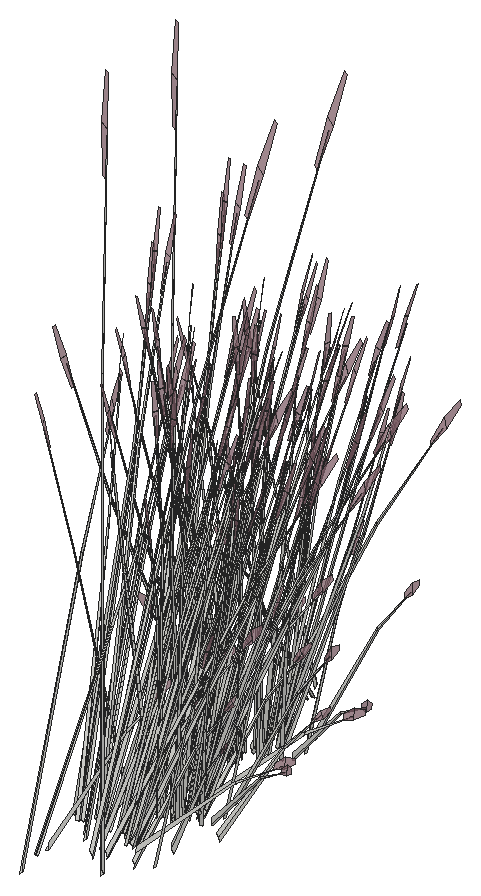
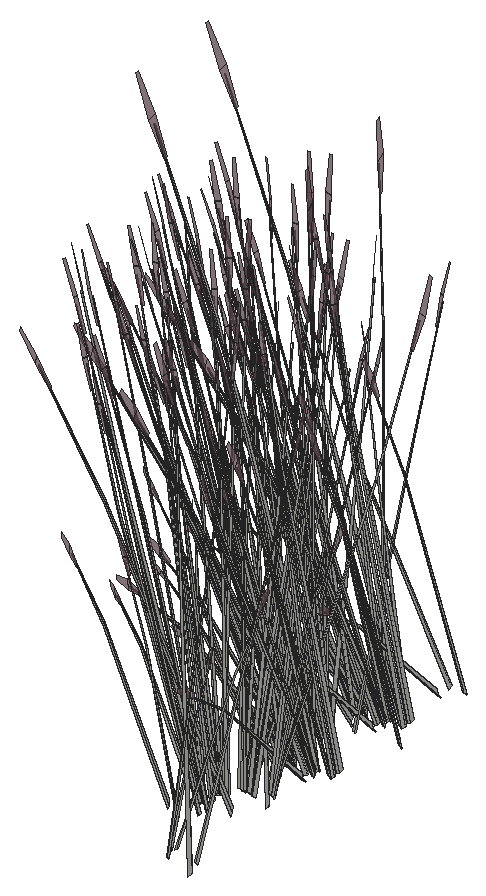
# SketchUp Ruby script. Lengths in inches.
U = 1.inch
M = Sketchup.active_model
def pt(a) = Geom::Point3d.new(a.map { |v| v * U })
def face(e, loops, mat)
  f = e.add_face(loops[0].map { |a| pt(a) })
  loops[1..].each { |l| e.add_face(l.map { |a| pt(a) }).erase! }
  f.material = f.back_material = mat if mat
  f
end
# faces: each face lists its corners as indices into pts; further lists are holes
def faces(e, pts, list, mat = nil) = list.each { |f| face(e, (f[0].is_a?(Array) ? f : [f]).map { |l| l.map { |i| pts[i] } }, mat) }
# xy, xz, yz: faces in a plane at the given z, y or x. An outline is a flat list of corners, or four numbers for a rectangle; further outlines are holes
def ring(l) = l.size == 4 ? [[l[0], l[1]], [l[2], l[1]], [l[2], l[3]], [l[0], l[3]]] : l.each_slice(2).to_a
def flat(e, list, mat, &to3) = list.each { |f| face(e, (f[0].is_a?(Array) ? f : [f]).map { |l| ring(l).map { |u, v| to3.(u, v) } }, mat) }
def xy(e, z, list, mat = nil) = flat(e, list, mat) { |x, y| [x, y, z] }
def xz(e, y, list, mat = nil) = flat(e, list, mat) { |x, z| [x, y, z] }
def yz(e, x, list, mat = nil) = flat(e, list, mat) { |y, z| [x, y, z] }
def lines(e, pts, list) = list.each { |a, b| e.add_line(pt(pts[a]), pt(pts[b])) }
# prism: a flat outline (further loops are holes) pulled along v
def prism(e, loops, v, mat = nil)
  f = face(e, loops, mat); d = Geom::Vector3d.new(v.map { |x| x * U })
  f.pushpull(f.normal.samedirection?(d) ? d.length : -d.length)
end
def box(e, o, s, mat = nil) = prism(e, [[o, [o[0] + s[0], o[1], o[2]], [o[0] + s[0], o[1] + s[1], o[2]], [o[0], o[1] + s[1], o[2]]]], [0, 0, s[2]], mat)
def at(x, y, z, deg = 0) = Geom::Transformation.translation(pt([x, y, z])) * Geom::Transformation.rotation(ORIGIN, Z_AXIS, deg.degrees)
def axes(o, x, y, z) = Geom::Transformation.new([*x, 0, *y, 0, *z, 0, *pt(o).to_a, 1])
def part(name) = M.definitions.add(name)
# library, detail: a bought-in or finely detailed component or shape, given as its bounding box
def library(name, o, s) = part(name).tap { |d| box(d.entities, o, s) }
def detail(e, o, s) = box(e.add_group.entities, o, s)
def put(e, d, t, mat = nil) = e.add_instance(d, t).tap { |i| i.material = mat if mat }
def group(e, t, mat = nil) = e.add_group.tap { |g| g.transformation = t; g.material = mat if mat }.entities
root = M.entities
M.materials.add("LightPink_Translucent").color = [144, 107, 117]
M.materials["LightPink_Translucent"].alpha = 0.75
c1 = part("blade")
p = [[2.15,0.21,22],[0,0.17,0],[0.09,0.45,0],[2.18,0.31,22],[2.29,0.31,22],[0.38,0.45,0],
  [2.48,0.24,33],[2.49,0.24,33],[2.48,0.22,33]]
faces(c1.entities,p,[[0,1,2,3],[4,5,2,3],[6,3,4,7],[8,0,3,6]])
c2 = part("seeds")
p = [[0.3,-0.1,1.38],[-0.01,-0.03,1.59],[-0.01,-0.03,0.03],[0.14,-0.07,-0.07],[0.29,-0.03,3],[0.15,0.01,3.11]]
faces(c2.entities,p,[[0,1,2,3],[1,0,4,5]],"LightPink_Translucent")
c3 = part("blade with seeds")
put(c3.entities,c1,at(0,0,0))
put(c3.entities,c2,axes([2.4,0.25,30.99],[1.5799,-0.05474,1.17369],[-0.12525,1.92788,0.29478],[-0.07173,-0.02425,1.56792]))
put(root,c3,axes([691.71,317.27,267.26],[-0.12452,-0.47997,-0.02898],[0.58854,-0.11034,-0.1314],[0.1229,0.03043,0.43341]))
put(root,c3,axes([690.1875,317.26,268.18],[0.03484,-0.58066,-0.10093],[0.65957,0.01587,-0.56021],[0.25402,0.04034,0.85122]))
put(root,c3,axes([690.09,317.03,268.19],[-0.37017,-0.35748,0.29394],[0.42268,-0.3384,-0.37948],[0.21476,0.05149,0.72609]))
put(root,c3,axes([686.65,312.02,267.22],[-0.01592,-0.21915,1.42242],[0.69015,0.14538,0.11501],[-0.04269,0.3123,0.60807]))
put(root,c3,axes([688.15,320.03,268.19],[-0.19614,0.43908,0.29394],[-0.57222,-0.12807,-0.37948],[-0.05247,-0.17678,0.72609]))
put(root,c3,axes([689.61,320.21,267.93],[0.46327,0.38957,0.39842],[-0.49199,0.33598,0.32852],[0.08546,-0.18277,0.82444]))
put(root,c3,axes([689.78,320.25,267.93],[0.53464,0.0266,0.05337],[-0.01466,0.40172,0.42015],[0.05594,-0.15388,0.64067]))
put(root,c3,axes([687.27,312.85,268.13],[0.31051,0.46426,-0.58968],[-0.63919,0.25873,0.07116],[0.07261,0.22432,0.83415]))
put(root,c3,axes([689.38,320.52,268.19],[-0.4402,0.30062,0.29394],[-0.41671,-0.34326,-0.37948],[0.0634,-0.1744,0.72609]))
put(root,c3,axes([690.16,321.33,268.13],[0.33983,-0.45051,-0.58968],[0.59551,0.32017,0.07116],[0.20291,-0.16322,0.83415]))
put(root,c3,axes([690.14,321.12,267.89],[-0.16713,-0.52135,-0.42412],[0.63294,-0.0912,-0.32852],[0.18138,-0.14003,0.81151]))
put(root,c3,axes([686.8,314.02,267.91],[0.08247,0.09194,1.45204],[0.66552,0.03612,-0.22964],[0.06692,0.20277,0.11645]))
put(root,c3,axes([690.76,316.91,267.91],[0.13956,-0.00966,1.45204],[0.38281,-0.44358,-0.22964],[0.24825,0.05855,0.11645]))
put(root,c3,axes([690.44,321.5,268.18],[-0.60181,-0.31483,-0.10093],[0.34671,-0.45593,-0.56021],[0.17003,-0.15849,0.85122]))
put(root,c3,axes([690.22,316.98,268.13],[0.65035,0.01375,-0.58968],[-0.04368,0.5789,0.07116],[0.27552,0.06109,0.83415]))
put(root,c3,axes([691.92,321.36,267.91],[-0.08498,-0.00434,1.47228],[-0.35287,-0.46464,-0.13912],[0.14171,-0.15278,0.26054]))
put(root,c3,axes([690.92,320.09,266.3],[-0.2167,0.29065,0.95334],[-0.18626,-0.3905,0.70045],[0.17898,-0.09785,0.20998]))
put(root,c3,axes([690.61,317.22,267.76],[0.37017,0.35748,-0.29394],[-0.42268,0.3384,0.37948],[0.21476,0.05149,0.72609]))
put(root,c3,axes([690.42,317.35,267.93],[-0.03276,0.43418,0.05337],[-0.49468,-0.0119,0.42015],[0.18949,0.04543,0.64067]))
put(root,c3,axes([690.61,321.18,267.76],[0.56631,-0.0816,-0.29394],[0.14954,0.46647,0.37948],[0.16229,-0.12529,0.72609]))
put(root,c3,axes([690.47,317.22,267.93],[-0.47971,0.37622,0.39842],[-0.41372,-0.39954,0.32852],[0.22506,0.0694,0.82444]))
put(root,c3,axes([690.15,321.45,268.19],[-0.56631,0.0816,0.29394],[-0.14954,-0.46647,-0.37948],[0.16229,-0.12529,0.72609]))
put(root,c3,axes([688.94,317.65,268.19],[-0.10048,-0.4599,0.29394],[0.5744,-0.12144,-0.37948],[0.15428,0.13179,0.72609]))
put(root,c3,axes([689.28,316.3,267.22],[-0.24166,-0.09837,1.42242],[0.50011,-0.41269,0.11501],[0.3117,0.18617,0.60807]))
put(root,c3,axes([689.33,315.01,267.71],[-0.56218,-0.29666,1.14775],[0.59361,-0.46189,0.49522],[0.18138,0.27836,1.10941]))
put(root,c3,axes([690.18,317.42,266.3],[-0.36631,-0.16417,0.95334],[0.47299,-0.16681,0.70045],[0.12758,0.1413,0.20998]))
put(root,c3,axes([688.89,317.89,268.18],[0.38768,-0.48872,-0.10093],[0.56143,0.28156,-0.56021],[0.19516,0.13808,0.85122]))
put(root,c3,axes([690.66,321.38,267.93],[0.44663,0.24013,0.05337],[-0.26003,0.34195,0.42015],[0.14319,-0.11055,0.64067]))
put(root,c3,axes([690.54,321.28,267.93],[0.16135,0.52549,0.39842],[-0.63294,0.0912,0.32852],[0.18654,-0.12359,0.82444]))
put(root,c3,axes([692.24,321.91,267.91],[0.09028,-0.08697,1.45204],[-0.11555,-0.53348,-0.22964],[0.22652,-0.10115,0.11645]))
put(root,c3,axes([686.33,317.23,268.19],[0.4402,-0.30062,0.29394],[0.41671,0.34326,-0.37948],[-0.0634,0.1744,0.72609]))
put(root,c3,axes([688.38,318.29,267.91],[0.00193,-0.06913,1.47228],[0.55753,-0.30498,-0.13912],[0.19366,0.10886,0.26054]))
put(root,c3,axes([689.28,315.57,266.36],[-0.01777,-0.53759,1.17256],[0.80434,0.13935,0.49647],[-0.19024,0.29416,1.1068]))
put(root,c3,axes([689.35,317.65,267.89],[0.64198,-0.13573,-0.42412],[0.1123,0.514,-0.32852],[0.17243,0.1473,0.81151]))
put(root,c3,axes([687.57,317.72,268.19],[0.19614,-0.43908,0.29394],[0.57222,0.12807,-0.37948],[0.05247,0.17678,0.72609]))
put(root,c3,axes([689.03,318.07,267.93],[-0.29569,0.36271,0.05337],[-0.42107,-0.21117,0.42015],[0.13613,0.11629,0.64067]))
put(root,c3,axes([690.47,322.72,268.18],[-0.32734,-0.51701,-0.10093],[0.58097,-0.25407,-0.56021],[0.24483,-0.06821,0.85122]))
put(root,c3,axes([690.4375,322.28,267.89],[0.17625,-0.51936,-0.42412],[0.60429,0.17802,-0.32852],[0.2433,-0.04762,0.81151]))
put(root,c3,axes([688.34,319.29,268.6875],[0.44958,-0.32756,-0.05385],[0.41194,0.35875,-0.24415],[0.029,0.10165,0.8053]))
put(root,c3,axes([689.16,317.97,267.93],[-0.64708,0.13103,0.39842],[-0.1123,-0.514,0.32852],[0.15218,0.15149,0.82444]))
put(root,c3,axes([690.32,322.47,268.13],[0.57168,-0.25217,-0.58968],[0.3186,0.51908,0.07116],[0.27622,-0.05897,0.83415]))
put(root,c3,axes([687.39,318.12,267.93],[-0.47939,0.19405,0.05337],[-0.23464,-0.35385,0.42015],[0.0463,0.15598,0.64067]))
put(root,c3,axes([686.05,317.3125,268.48],[0.71502,0.02829,-0.11203],[-0.01954,0.53563,-0.62183],[-0.04967,0.20629,0.94486]))
put(root,c3,axes([687.375,317.91,268.18],[0.63664,-0.26583,-0.10093],[0.31286,0.47181,-0.56021],[0.084,0.19882,0.85122]))
put(root,c3,axes([687.5625,318.08,268.2],[-0.64106,-0.14927,0.44225],[0.21921,-0.49074,0.36465],[0.03852,0.19299,0.91512]))
put(root,c3,axes([690.24,322.57,268.19],[-0.54068,-0.15928,0.29394],[0.1577,-0.46469,-0.37948],[0.21769,-0.04261,0.72609]))
put(root,c3,axes([686.54,317.51,268.15],[0.46573,0.38364,-0.47077],[-0.49199,0.33598,-0.36465],[-0.07086,0.19492,0.90078]))
put(root,c3,axes([687.92,317.89,267.89],[0.63954,0.14313,-0.42412],[-0.21921,0.49074,-0.32852],[0.05864,0.19758,0.81151]))
put(root,c3,axes([688.29,316.87,267.22],[-0.14872,-0.18332,1.42242],[0.6872,-0.15433,0.11501],[0.15531,0.28779,0.60807]))
put(root,c3,axes([687.63,318.1875,267.76],[-0.19614,0.43908,-0.29394],[-0.57222,-0.12807,0.37948],[0.05247,0.17678,0.72609]))
put(root,c3,axes([690.81,322.52,267.76],[0.54068,0.15928,-0.29394],[-0.1577,0.46469,0.37948],[0.21769,-0.04261,0.72609]))
put(root,c3,axes([687.07,316.96,267.22],[-0.01592,-0.21915,1.42242],[0.69015,0.14538,0.11501],[-0.04269,0.3123,0.60807]))
put(root,c3,axes([689.34,321.94,267.22],[-0.26985,0.01293,1.42242],[0.17902,-0.56047,0.11501],[0.38456,0.03467,0.60807]))
put(root,c3,axes([687.69,317.79,268.13],[0.31051,0.46426,-0.58968],[-0.63919,0.25873,0.07116],[0.07261,0.22432,0.83415]))
put(root,c3,axes([690.73,322.71,267.93],[0.23895,0.38931,0.05337],[-0.43573,0.19055,0.42015],[0.19208,-0.0376,0.64067]))
put(root,c3,axes([690.68,322.57,267.93],[-0.18381,0.5206,0.39842],[-0.60429,-0.17802,0.32852],[0.23764,-0.03129,0.82444]))
put(root,c3,axes([687.23,318.96,267.91],[0.08247,0.09194,1.45204],[0.66552,0.03612,-0.22964],[0.06692,0.20277,0.11645]))
put(root,c3,axes([691.96,322.61,266.3],[-0.40197,0.09426,0.95334],[0.18921,-0.38956,0.70045],[0.21325,0.02666,0.20998]))
put(root,c3,axes([686.97,328.16,268.13],[-0.31051,-0.46426,-0.58968],[0.63919,-0.25873,0.07116],[-0.07261,-0.22432,0.83415]))
put(root,c3,axes([686.16,318.08,266.79],[0.01429,-0.29475,1.28107],[0.64291,0.15569,0.17703],[-0.0557,0.31414,0.60492]))
put(root,c3,axes([691.77,324.26,267.91],[-0.05883,-0.04999,1.47228],[0.12868,-0.53581,-0.13912],[0.23172,-0.03423,0.26054]))
put(root,c3,axes([691.26,323.8125,267.26],[-0.12452,-0.47997,-0.02898],[0.58854,-0.11034,-0.1314],[0.1229,0.03043,0.43341]))
put(root,c3,axes([689.73,323.8,268.18],[0.03484,-0.58066,-0.10093],[0.65957,0.01587,-0.56021],[0.25402,0.04034,0.85122]))
put(root,c3,axes([688.27,328.61,268.13],[0.01693,-0.52814,-0.58968],[0.71285,0.03547,0.07116],[0.07523,-0.22375,0.83415]))
put(root,c3,axes([689.63,323.57,268.19],[-0.37017,-0.35748,0.29394],[0.42268,-0.3384,-0.37948],[0.21476,0.05149,0.72609]))
put(root,c3,axes([689.26,327.79,267.91],[-0.00628,-0.11364,1.45204],[-0.53042,-0.32843,-0.22964],[0.08201,-0.19909,0.11645]))
put(root,c3,axes([687.03,327.77,267.76],[0.19614,-0.43908,-0.29394],[0.57222,0.12807,0.37948],[-0.05247,-0.17678,0.72609]))
put(root,c3,axes([687.46,328.35,267.22],[-0.12114,0.19625,1.42242],[-0.50818,-0.40613,0.11501],[0.22925,-0.25313,0.60807]))
put(root,c3,axes([689.12,327.38,267.91],[-0.06607,0.04361,1.47228],[-0.64734,-0.14714,-0.13912],[-0.02343,-0.19032,0.26054]))
put(root,c3,axes([688.12,328.4375,267.89],[-0.46573,-0.38364,-0.42412],[0.49199,-0.33598,-0.32852],[0.07086,-0.19492,0.81151]))
put(root,c3,axes([690.3,323.45,267.91],[0.13956,-0.00966,1.45204],[0.38281,-0.44358,-0.22964],[0.24825,0.05855,0.11645]))
put(root,c3,axes([687.1,327.87,267.93],[0.64106,0.14927,0.39842],[-0.21921,0.49074,0.32852],[-0.03852,-0.19299,0.82444]))
put(root,c3,axes([688.61,328.64,268.18],[-0.71502,-0.02829,-0.10093],[0.01954,-0.53563,-0.56021],[0.04967,-0.20629,0.85122]))
put(root,c3,axes([689.76,323.52,268.13],[0.65035,0.01375,-0.58968],[-0.04368,0.5789,0.07116],[0.27552,0.06109,0.83415]))
put(root,c3,axes([688.56,328.3,267.76],[0.4402,-0.30062,-0.29394],[0.41671,0.34326,0.37948],[0.0634,-0.1744,0.72609]))
put(root,c3,axes([687.27,327.83,267.93],[0.47939,-0.19405,0.05337],[0.23464,0.35385,0.42015],[-0.0463,-0.15598,0.64067]))
put(root,c3,axes([690.16,323.76,267.76],[0.37017,0.35748,-0.29394],[-0.42268,0.3384,0.37948],[0.21476,0.05149,0.72609]))
put(root,c3,axes([689.97,323.89,267.93],[-0.03276,0.43418,0.05337],[-0.49468,-0.0119,0.42015],[0.18949,0.04543,0.64067]))
put(root,c3,axes([690.01,323.76,267.93],[-0.47971,0.37622,0.39842],[-0.41372,-0.39954,0.32852],[0.22506,0.0694,0.82444]))
put(root,c3,axes([687.09,328.23,268.19],[-0.19614,0.43908,0.29394],[-0.57222,-0.12807,-0.37948],[-0.05247,-0.17678,0.72609]))
put(root,c3,axes([688.56,328.41,267.93],[0.46327,0.38957,0.39842],[-0.49199,0.33598,0.32852],[0.08546,-0.18277,0.82444]))
put(root,c3,axes([688.73,328.45,267.93],[0.53464,0.0266,0.05337],[-0.01466,0.40172,0.42015],[0.05594,-0.15388,0.64067]))
put(root,c3,axes([688.49,324.19,268.19],[-0.10048,-0.4599,0.29394],[0.5744,-0.12144,-0.37948],[0.15428,0.13179,0.72609]))
put(root,c3,axes([688.33,328.72,268.19],[-0.4402,0.30062,0.29394],[-0.41671,-0.34326,-0.37948],[0.0634,-0.1744,0.72609]))
put(root,c3,axes([688.83,322.84,267.22],[-0.24166,-0.09837,1.42242],[0.50011,-0.41269,0.11501],[0.3117,0.18617,0.60807]))
put(root,c3,axes([689.11,329.53,268.13],[0.33983,-0.45051,-0.58968],[0.59551,0.32017,0.07116],[0.20291,-0.16322,0.83415]))
put(root,c3,axes([689.09,329.32,267.89],[-0.16713,-0.52135,-0.42412],[0.63294,-0.0912,-0.32852],[0.18138,-0.14003,0.81151]))
put(root,c3,axes([688.87,321.55,267.71],[-0.56218,-0.29666,1.14775],[0.59361,-0.46189,0.49522],[0.18138,0.27836,1.10941]))
put(root,c3,axes([689.72,323.96,266.3],[-0.36631,-0.16417,0.95334],[0.47299,-0.16681,0.70045],[0.12758,0.1413,0.20998]))
put(root,c3,axes([689.39,329.7,268.18],[-0.60181,-0.31483,-0.10093],[0.34671,-0.45593,-0.56021],[0.17003,-0.15849,0.85122]))
put(root,c3,axes([688.43,324.43,268.18],[0.38768,-0.48872,-0.10093],[0.56143,0.28156,-0.56021],[0.19516,0.13808,0.85122]))
put(root,c3,axes([685.88,323.77,268.19],[0.4402,-0.30062,0.29394],[0.41671,0.34326,-0.37948],[-0.0634,0.1744,0.72609]))
put(root,c3,axes([687.93,324.84,267.91],[0.00193,-0.06913,1.47228],[0.55753,-0.30498,-0.13912],[0.19366,0.10886,0.26054]))
put(root,c3,axes([690.87,329.56,267.91],[-0.08498,-0.00434,1.47228],[-0.35287,-0.46464,-0.13912],[0.14171,-0.15278,0.26054]))
put(root,c3,axes([688.83,322.11,266.36],[-0.01777,-0.53759,1.17256],[0.80434,0.13935,0.49647],[-0.19024,0.29416,1.1068]))
put(root,c3,axes([688.89,324.1875,267.89],[0.64198,-0.13573,-0.42412],[0.1123,0.514,-0.32852],[0.17243,0.1473,0.81151]))
put(root,c3,axes([687.11,324.26,268.19],[0.19614,-0.43908,0.29394],[0.57222,0.12807,-0.37948],[0.05247,0.17678,0.72609]))
put(root,c3,axes([689.56,329.38,267.76],[0.56631,-0.0816,-0.29394],[0.14954,0.46647,0.37948],[0.16229,-0.12529,0.72609]))
put(root,c3,axes([688.58,324.61,267.93],[-0.29569,0.36271,0.05337],[-0.42107,-0.21117,0.42015],[0.13613,0.11629,0.64067]))
put(root,c3,axes([687.88,325.83,268.6875],[0.44958,-0.32756,-0.05385],[0.41194,0.35875,-0.24415],[0.029,0.10165,0.8053]))
put(root,c3,axes([688.7,324.51,267.93],[-0.64708,0.13103,0.39842],[-0.1123,-0.514,0.32852],[0.15218,0.15149,0.82444]))
put(root,c3,axes([689.09,329.65,268.19],[-0.56631,0.0816,0.29394],[-0.14954,-0.46647,-0.37948],[0.16229,-0.12529,0.72609]))
put(root,c3,axes([686.93,324.66,267.93],[-0.47939,0.19405,0.05337],[-0.23464,-0.35385,0.42015],[0.0463,0.15598,0.64067]))
put(root,c3,axes([685.6,323.85,268.48],[0.71502,0.02829,-0.11203],[-0.01954,0.53563,-0.62183],[-0.04967,0.20629,0.94486]))
put(root,c3,axes([686.92,324.45,268.18],[0.63664,-0.26583,-0.10093],[0.31286,0.47181,-0.56021],[0.084,0.19882,0.85122]))
put(root,c3,axes([687.1,324.625,268.2],[-0.64106,-0.14927,0.44225],[0.21921,-0.49074,0.36465],[0.03852,0.19299,0.91512]))
put(root,c3,axes([689.61,329.58,267.93],[0.44663,0.24013,0.05337],[-0.26003,0.34195,0.42015],[0.14319,-0.11055,0.64067]))
put(root,c3,axes([689.48,329.48,267.93],[0.16135,0.52549,0.39842],[-0.63294,0.0912,0.32852],[0.18654,-0.12359,0.82444]))
put(root,c3,axes([691.1875,330.11,267.91],[0.09028,-0.08697,1.45204],[-0.11555,-0.53348,-0.22964],[0.22652,-0.10115,0.11645]))
put(root,c3,axes([686.09,324.05,268.15],[0.46573,0.38364,-0.47077],[-0.49199,0.33598,-0.36465],[-0.07086,0.19492,0.90078]))
put(root,c3,axes([687.47,324.43,267.89],[0.63954,0.14313,-0.42412],[-0.21921,0.49074,-0.32852],[0.05864,0.19758,0.81151]))
put(root,c3,axes([687.83,323.41,267.22],[-0.14872,-0.18332,1.42242],[0.6872,-0.15433,0.11501],[0.15531,0.28779,0.60807]))
put(root,c3,axes([687.18,324.73,267.76],[-0.19614,0.43908,-0.29394],[-0.57222,-0.12807,0.37948],[0.05247,0.17678,0.72609]))
put(root,c3,axes([686.62,323.5,267.22],[-0.01592,-0.21915,1.42242],[0.69015,0.14538,0.11501],[-0.04269,0.3123,0.60807]))
put(root,c3,axes([689.41,330.92,268.18],[-0.32734,-0.51701,-0.10093],[0.58097,-0.25407,-0.56021],[0.24483,-0.06821,0.85122]))
put(root,c3,axes([689.38,330.48,267.89],[0.17625,-0.51936,-0.42412],[0.60429,0.17802,-0.32852],[0.2433,-0.04762,0.81151]))
put(root,c3,axes([687.23,324.33,268.13],[0.31051,0.46426,-0.58968],[-0.63919,0.25873,0.07116],[0.07261,0.22432,0.83415]))
put(root,c3,axes([686.77,325.51,267.91],[0.08247,0.09194,1.45204],[0.66552,0.03612,-0.22964],[0.06692,0.20277,0.11645]))
put(root,c3,axes([689.27,330.67,268.13],[0.57168,-0.25217,-0.58968],[0.3186,0.51908,0.07116],[0.27622,-0.05897,0.83415]))
put(root,c3,axes([689.18,330.77,268.19],[-0.54068,-0.15928,0.29394],[0.1577,-0.46469,-0.37948],[0.21769,-0.04261,0.72609]))
put(root,c3,axes([689.75,330.72,267.76],[0.54068,0.15928,-0.29394],[-0.1577,0.46469,0.37948],[0.21769,-0.04261,0.72609]))
put(root,c3,axes([688.28,330.14,267.22],[-0.26985,0.01293,1.42242],[0.17902,-0.56047,0.11501],[0.38456,0.03467,0.60807]))
put(root,c3,axes([689.67,330.91,267.93],[0.23895,0.38931,0.05337],[-0.43573,0.19055,0.42015],[0.19208,-0.0376,0.64067]))
put(root,c3,axes([689.63,330.77,267.93],[-0.18381,0.5206,0.39842],[-0.60429,-0.17802,0.32852],[0.23764,-0.03129,0.82444]))
put(root,c3,axes([690.71,332.46,267.91],[-0.05883,-0.04999,1.47228],[0.12868,-0.53581,-0.13912],[0.23172,-0.03423,0.26054]))
put(root,c3,axes([690.2,332.01,267.26],[-0.12452,-0.47997,-0.02898],[0.58854,-0.11034,-0.1314],[0.1229,0.03043,0.43341]))
put(root,c3,axes([688.68,332,268.18],[0.03484,-0.58066,-0.10093],[0.65957,0.01587,-0.56021],[0.25402,0.04034,0.85122]))
put(root,c3,axes([686.93,336.8,268.13],[0.01693,-0.52814,-0.58968],[0.71285,0.03547,0.07116],[0.07523,-0.22375,0.83415]))
put(root,c3,axes([688.58,331.77,268.19],[-0.37017,-0.35748,0.29394],[0.42268,-0.3384,-0.37948],[0.21476,0.05149,0.72609]))
put(root,c3,axes([687.92,335.98,267.91],[-0.00628,-0.11364,1.45204],[-0.53042,-0.32843,-0.22964],[0.08201,-0.19909,0.11645]))
put(root,c3,axes([685.69,335.95,267.76],[0.19614,-0.43908,-0.29394],[0.57222,0.12807,0.37948],[-0.05247,-0.17678,0.72609]))
put(root,c3,axes([686.125,336.54,267.22],[-0.12114,0.19625,1.42242],[-0.50818,-0.40613,0.11501],[0.22925,-0.25313,0.60807]))
put(root,c3,axes([687.78,335.57,267.91],[-0.06607,0.04361,1.47228],[-0.64734,-0.14714,-0.13912],[-0.02343,-0.19032,0.26054]))
